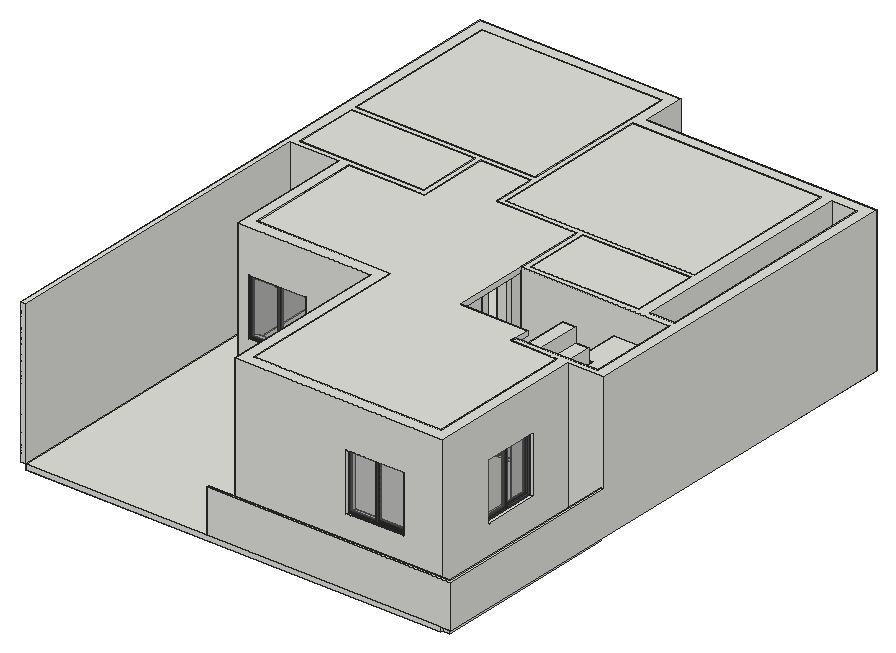
# SketchUp Ruby script. Lengths in inches.
U = 1.inch
M = Sketchup.active_model
def pt(a) = Geom::Point3d.new(a.map { |v| v * U })
def face(e, loops, mat)
  f = e.add_face(loops[0].map { |a| pt(a) })
  loops[1..].each { |l| e.add_face(l.map { |a| pt(a) }).erase! }
  f.material = f.back_material = mat if mat
  f
end
# faces: each face lists its corners as indices into pts; further lists are holes
def faces(e, pts, list, mat = nil) = list.each { |f| face(e, (f[0].is_a?(Array) ? f : [f]).map { |l| l.map { |i| pts[i] } }, mat) }
# xy, xz, yz: faces in a plane at the given z, y or x. An outline is a flat list of corners, or four numbers for a rectangle; further outlines are holes
def ring(l) = l.size == 4 ? [[l[0], l[1]], [l[2], l[1]], [l[2], l[3]], [l[0], l[3]]] : l.each_slice(2).to_a
def flat(e, list, mat, &to3) = list.each { |f| face(e, (f[0].is_a?(Array) ? f : [f]).map { |l| ring(l).map { |u, v| to3.(u, v) } }, mat) }
def xy(e, z, list, mat = nil) = flat(e, list, mat) { |x, y| [x, y, z] }
def xz(e, y, list, mat = nil) = flat(e, list, mat) { |x, z| [x, y, z] }
def yz(e, x, list, mat = nil) = flat(e, list, mat) { |y, z| [x, y, z] }
def lines(e, pts, list) = list.each { |a, b| e.add_line(pt(pts[a]), pt(pts[b])) }
# prism: a flat outline (further loops are holes) pulled along v
def prism(e, loops, v, mat = nil)
  f = face(e, loops, mat); d = Geom::Vector3d.new(v.map { |x| x * U })
  f.pushpull(f.normal.samedirection?(d) ? d.length : -d.length)
end
def box(e, o, s, mat = nil) = prism(e, [[o, [o[0] + s[0], o[1], o[2]], [o[0] + s[0], o[1] + s[1], o[2]], [o[0], o[1] + s[1], o[2]]]], [0, 0, s[2]], mat)
def at(x, y, z, deg = 0) = Geom::Transformation.translation(pt([x, y, z])) * Geom::Transformation.rotation(ORIGIN, Z_AXIS, deg.degrees)
def axes(o, x, y, z) = Geom::Transformation.new([*x, 0, *y, 0, *z, 0, *pt(o).to_a, 1])
def part(name) = M.definitions.add(name)
# library, detail: a bought-in or finely detailed component or shape, given as its bounding box
def library(name, o, s) = part(name).tap { |d| box(d.entities, o, s) }
def detail(e, o, s) = box(e.add_group.entities, o, s)
def put(e, d, t, mat = nil) = e.add_instance(d, t).tap { |i| i.material = mat if mat }
def group(e, t, mat = nil) = e.add_group.tap { |g| g.transformation = t; g.material = mat if mat }.entities
root = M.entities
M.materials.add("[0099_LightSteelBlue]").color = [176, 196, 222]
M.materials.add("[0135_DarkGray]").color = [81, 81, 81]
M.materials.add("[Translucent Glass Gray]1").color = [128, 128, 128]
M.materials["[Translucent Glass Gray]1"].alpha = 0.15
M.materials.add("[Wood Bamboo]").color = [112, 66, 27]
c1 = library("door58",[0,0,0],[34.0625,4.69,78.29])
c2 = library("Flush door assembly",[0,-5.12,-0.12],[5.12,39.07,81.6])
c3 = library("WP_2073",[15.29,-17.35,0],[14.73,29.14,28.74])
c4 = library("Shower-Trim-Delta-Modern-Monitor_14S_Shower_Trim-T14267-PP",[-3.32,-7.77,-3.94],[6.64,7.77,30.2])
c5 = part("PENTEK_RP Fineline 50S_Sliding_DoorCase_E1")
box(c5.entities,[0,0,0],[1.51,3.66,99.27],"[0135_DarkGray]")
c6 = part("PENTEK_RP Fineline 50S_SlidingDooe_Case_E2")
box(c6.entities,[0,0,0],[96.25,3.66,1.51],"[0135_DarkGray]")
c7 = part("pentek_RP Fineline 50S_SlidingDoor_Case")
put(c7.entities,c5,at(97.76,0,0))
put(c7.entities,c6,at(1.51,0,0))
put(c7.entities,c5,at(0,0,0))
put(c7.entities,c6,at(1.51,0,97.76))
c8 = part("PENTEK_RP Fineline 50S_SlidingDoor_GlazingBead_2")
box(c8.entities,[0,0,0],[0.56,0.59,94.39],"[0135_DarkGray]")
c9 = part("PENTEK_RP Fineline 50S_SlidingDoor_Glass")
box(c9.entities,[0,0,0],[46.58,0.16,94.39],"[Translucent Glass Gray]1")
c10 = part("PENTEK_RP Fineline 50S_SlidingDoor_GlazingBead")
box(c10.entities,[0,0,0],[45.47,0.59,0.56],"[0135_DarkGray]")
c11 = part("PENTEK_RP Fineline 50S_SlidingDoor_Leaf_E1")
prism(c11.entities,[[[0,1.97,0],[1.49,1.97,0],[1.49,1.57,0],[0.93,1.57,0],[0.93,0,0],[0,0,0]]],[0,0,96.25],"[0135_DarkGray]")
c12 = part("PENTEK_RP Fineline 50S_SlidingDoor_Leaf_E2")
xy(c12.entities,0,[[0,0,0,1.57,0.56,1.57,0.56,1.97,46.02,1.97,46.02,1.57,46.58,1.57,46.58,0]],"[0135_DarkGray]")
xy(c12.entities,0.93,[[0,0,46.58,1.57]],"[0135_DarkGray]")
xy(c12.entities,1.49,[[0.56,1.57,46.02,1.97]],"[0135_DarkGray]")
xz(c12.entities,0,[[0,0,46.58,0.93]],"[0135_DarkGray]")
xz(c12.entities,1.57,[[0,0,0.56,0.93],[46.02,0,46.58,0.93],[0.56,0.93,46.02,1.49]],"[0135_DarkGray]")
xz(c12.entities,1.97,[[0.56,0,46.02,1.49]],"[0135_DarkGray]")
yz(c12.entities,0,[[0,0,1.57,0.93]],"[0135_DarkGray]")
yz(c12.entities,0.56,[[1.57,0,1.97,1.49]],"[0135_DarkGray]")
yz(c12.entities,46.02,[[1.57,0,1.97,1.49]],"[0135_DarkGray]")
yz(c12.entities,46.58,[[0,0,1.57,0.93]],"[0135_DarkGray]")
c13 = part("PENTEK_RP Fineline S_SlidingDoor_Leaf1")
put(c13.entities,c8,at(0.93,0,0.93))
put(c13.entities,c8,at(46.96,0,0.93))
put(c13.entities,c9,at(1.49,1.42,0.93))
put(c13.entities,c10,at(1.49,0,0.93))
put(c13.entities,c9,at(1.49,0.59,0.93))
put(c13.entities,c11,at(0,0,0))
put(c13.entities,c11,axes([48.44,0,0],[-1,0,0],[0,1,0],[0,0,1]))
put(c13.entities,c12,axes([0.93,0,96.25],[1,0,0],[0,1,0],[0,0,-1]))
put(c13.entities,c12,at(0.93,0,0))
put(c13.entities,c10,at(1.49,0,94.77))
c14 = part("PENTEK_RP Fineline 50S_SlidingDoor_Leaf2")
put(c14.entities,c9,at(1.49,1.42,0.93))
put(c14.entities,c10,at(1.49,0,94.77))
put(c14.entities,c8,at(46.96,0,0.93))
put(c14.entities,c9,at(1.49,0.59,0.93))
put(c14.entities,c8,at(0.93,0,0.93))
put(c14.entities,c11,at(0,0,0))
put(c14.entities,c11,axes([48.44,0,0],[-1,0,0],[0,1,0],[0,0,1]))
put(c14.entities,c10,at(1.49,0,0.93))
put(c14.entities,c12,axes([0.93,0,96.25],[1,0,0],[0,1,0],[0,0,-1]))
put(c14.entities,c12,at(0.93,0,0))
c15 = part("PENTEK_RP+Fineline+50S_Sliding_Door+(1)")
put(c15.entities,c7,at(0,-1.88,-0.09))
put(c15.entities,c13,at(1.51,-2.27,1.42))
put(c15.entities,c14,at(49.32,-0.3,1.42))
c16 = part("Component\#1")
box(c16.entities,[0,0,0],[16.1,26,0.8])
c17 = part("Component\#2")
box(c17.entities,[0,0,0],[25.87,9.8,0.8])
c18 = part("Component\#3")
box(c18.entities,[0,0,0],[12.93,26,0.8])
c19 = library("Group69",[-16.93,-10.04,-8.23],[33.86,20.08,21.73])
c20 = part("Component\#4")
box(c20.entities,[0,0,0],[13.7,49,0.8])
c21 = part("Component\#5")
box(c21.entities,[0,0,0],[15.4,32.2,0.8])
c22 = part("Component\#6")
box(c22.entities,[0,0,0],[23.2,26,0.8],"[0099_LightSteelBlue]")
c23 = library("Group\#11",[-0.5,-0.5,-0.1],[125,90.5,0.2])
xy(root,-4,[[4.5,0,4.5,435,9,435,9,471,159,471,159,435,351,435,351,240,233,240,233,204,351,204,351,200,283,200,283,164,351,164,351,159.5,357.25,159.5,357.25,2.0625,351,2.0625,351,0]])
xy(root,0,[[4.5,0,4.5,435,9,435,9,471,159,471,159,435,351,435,351,240,227,240,227,204,315,204,315,200,293,200,293,164,351,164,351,159.5,357.25,159.5,357.25,2.0625,351,2.0625,351,0]])
xy(root,12,[[227,204,238,240]])
xy(root,24,[[238,204,249,240]])
xy(root,36,[[249,204,260,240]])
xy(root,48,[[260,204,271,240]])
xy(root,60,[[271,204,282,240]])
xy(root,72,[[282,204,293,240]])
xy(root,84,[[293,204,304,240]])
xy(root,96,[[315,164,351,164,351,240,304,240,304,204,315,204]])
xy(root,108,[[304,164,315,200]])
xy(root,120,[[293,164,304,200]])
xz(root,0,[[4.5,-4,351,0]])
xz(root,2.0625,[[351,-4,357.25,0]])
xz(root,159.5,[[351,-4,357.25,0]])
xz(root,164,[[283,-4,351,0],[293,0,351,0,351,96,315,96,315,108,304,108,304,120,293,120]])
xz(root,200,[[293,0,293,120,304,120,304,108,315,108,315,0]])
xz(root,204,[[227,0,315,0,315,96,304,96,304,84,293,84,293,72,282,72,282,60,271,60,271,48,260,48,260,36,249,36,249,24,238,24,238,12,227,12]])
xz(root,240,[[233,-4,351,0],[227,0,227,12,238,12,238,24,249,24,249,36,260,36,260,48,271,48,271,60,282,60,282,72,293,72,293,84,304,84,304,96,351,96,351,0]])
xz(root,435,[[4.5,-4,9,0],[159,-4,351,0]])
xz(root,471,[[9,-4,159,0]])
yz(root,4.5,[[0,-4,435,0]])
yz(root,9,[[435,-4,471,0]])
yz(root,159,[[435,-4,471,0]])
yz(root,227,[[204,0,240,12]])
yz(root,238,[[204,12,240,24]])
yz(root,249,[[204,24,240,36]])
yz(root,260,[[204,36,240,48]])
yz(root,271,[[204,48,240,60]])
yz(root,282,[[204,60,240,72]])
yz(root,293,[[164,0,200,120],[204,72,240,84]])
yz(root,304,[[204,84,240,96],[164,108,200,120]])
yz(root,315,[[200,0,204,96],[164,96,200,108]])
yz(root,351,[[0,-4,2.0625,0],[159.5,-4,164,0],[200,-4,204,96],[240,-4,435,0],[164,96,240,120]])
yz(root,357.25,[[2.0625,-4,159.5,0]])
put(root,c1,axes([156.6875,167,0],[0,-1.05686,0],[1,0,0],[0,0,1.02]))
put(root,c2,axes([111.88,288.7,0.12],[1,0,0],[0,0.81896,0],[0,0,0.98035]))
put(root,c3,axes([240.57,240.54,-0.55],[0.02117,0.99977,0.0026],[-0.83872,0.01765,0.04289],[0.05099,-0.00368,0.99869]))
put(root,c4,at(321,270.72,69.74,-90))
put(root,c3,axes([18.26,279.57,-0.55],[0.02117,0.99977,0.0026],[-0.83872,0.01765,0.04289],[0.05099,-0.00368,0.99869]))
put(root,c4,at(79.9,334.5,69.74))
put(root,c2,axes([262.8,297.88,0.12],[0,1,0],[-0.81896,0,0],[0,0,0.98035]))
put(root,c15,axes([249,32.69,36.04],[0.48352,0,0],[0,1,0],[0,0,0.48352]))
put(root,c15,axes([54,174.03,36.04],[0.48352,0,0],[0,1,0],[0,0,0.48352]))
put(root,c15,axes([325.32,123.5,36.04],[0,-0.48352,0],[1,0,0],[0,0,0.48352]))
g1 = group(root,at(54,180,0))
prism(g1,[[[25,25,0],[110,25,0],[110,0,0],[0,0,0],[0,96,0],[25,96,0]]],[0,0,4])
g2 = group(root,at(54,180,4))
prism(g2,[[[27,96,0],[27,27,0],[110,27,0],[110,0,0],[0,0,0],[0,96,0]],[[2.35,57.97,0],[21.91,57.97,0],[21.91,90.16,0],[2.35,90.16,0]]],[0,0,28])
put(g2,c16,axes([27,78.9,1],[0,1,0],[0,0,1],[1,0,0]))
put(g2,c16,axes([27,62,1],[0,1,0],[0,0,1],[1,0,0]))
put(g2,c16,axes([27,45.5,1],[0,1,0],[0,0,1],[1,0,0]))
put(g2,c16,axes([27,29,1],[0,1,0],[0,0,1],[1,0,0]))
put(g2,c17,axes([81.93,27,17.2],[-1,0,0],[0,0,1],[0,1,0]))
put(g2,c17,axes([81.93,27,6.8],[-1,0,0],[0,0,1],[0,1,0]))
put(g2,c18,axes([109,27,1],[-1,0,0],[0,0,1],[0,1,0]))
put(g2,c18,axes([95.27,27,1],[-1,0,0],[0,0,1],[0,1,0]))
put(g2,c18,axes([55.27,27,1],[-1,0,0],[0,0,1],[0,1,0]))
put(g2,c18,axes([41.93,27,1],[-1,0,0],[0,0,1],[0,1,0]))
g3 = group(g2,at(81.93,27,1))
box(g3,[-25.87,0,0],[25.87,0.8,5.2])
put(root,c19,at(65.87,254.12,30.8,90))
g4 = group(root,at(103,180,62))
box(g4,[0,0,0],[62,18,51])
put(g4,c20,axes([61,18,1],[-1,0,0],[0,0,1],[0,1,0]))
put(g4,c21,axes([46.7,18,17.8],[-1,0,0],[0,0,1],[0,1,0]))
put(g4,c20,axes([14.7,18,1],[-1,0,0],[0,0,1],[0,1,0]))
put(g4,c21,axes([30.7,18,17.8],[-1,0,0],[0,0,1],[0,1,0]))
g5 = group(g4,at(15.3,2,0),"[Wood Bamboo]")
xy(g5,2,[[2,0,29.4,16]])
xy(g5,15,[[2,0,29.4,16]])
xz(g5,0,[[2,2,29.4,15]])
xz(g5,16,[[[0,0,31.4,17],[2,2,29.4,15]]])
yz(g5,2,[[0,2,16,15]])
yz(g5,29.4,[[0,2,16,15]])
g6 = group(root,at(54,180,85))
box(g6,[0,0,0],[49,18,28])
put(g6,c22,axes([48,18,1],[-1,0,0],[0,0,1],[0,1,0]))
put(g6,c22,axes([24.2,18,1],[-1,0,0],[0,0,1],[0,1,0]))
g7 = group(root,at(9,38,120))
box(g7,[154.5,265,-4],[157.5,132,4])
box(g7,[0,301,-4],[150,132,4])
box(g7,[0,242.5,-4],[103.5,54,4])
box(g7,[222,206.5,-4],[90,54,4])
box(g7,[173,17,-6],[122,87.5,2])
xy(g7,-6,[[[156,0,312,121.5],[172,16,296,105.5]]])
xy(g7,-4,[[156,121.5,156,142,45,142,45,238,108,238,108,296.5,150,296.5,150,260.5,217.5,260.5,217.5,138.49,274,138.49,274,121.5]])
xy(g7,0,[[156,0,312,0,312,121.5,274,121.5,274,138.49,217.5,138.49,217.5,260.5,150,260.5,150,296.5,108,296.5,108,238,45,238,45,142,156,142]])
xz(g7,0,[[156,-6,312,0]])
xz(g7,16,[[172,-6,296,-4]])
xz(g7,105.5,[[172,-6,274,-4],[274,-6,296,-4]])
xz(g7,121.5,[[156,-6,274,-4],[274,-6,312,0]])
xz(g7,138.49,[[217.5,-4,274,0]])
xz(g7,142,[[45,-4,156,0]])
xz(g7,238,[[45,-4,108,0]])
xz(g7,260.5,[[150,-4,217.5,0]])
xz(g7,296.5,[[108,-4,150,0]])
yz(g7,45,[[142,-4,238,0]])
yz(g7,108,[[238,-4,296.5,0]])
yz(g7,150,[[260.5,-4,296.5,0]])
yz(g7,156,[[0,-6,0,0,142,0,142,-4,121.5,-4,121.5,-6]])
yz(g7,172,[[16,-6,105.5,-4]])
yz(g7,217.5,[[138.49,-4,260.5,0]])
yz(g7,274,[[121.5,-4,126,0],[126,-4,138.49,0]])
yz(g7,296,[[16,-6,105.5,-4]])
yz(g7,312,[[0,-6,121.5,0]])
put(g7,c23,at(172,16,-4))
g8 = group(root,at(0,0,0))
xy(g8,0,[[[0,0,0,480,168,480,168,444,360,444,360,0,156,0,156,2.0625,357.25,2.0625,357.25,159.5,330,159.5,330,29,156,29,156,131,165,131,165,38,321,38,321,159.5,282,159.5,282,164,351,164,351,200,222.1875,200,222.1875,204,351,204,351,240,226.5,240,226.5,298.5,203.5,298.5,203.5,303,235,303,235,298.5,231,298.5,231,244.5,321,244.5,321,298.5,267,298.5,267,303,321,303,321,435,163.5,435,163.5,303,167.5,303,167.5,298.5,159,298.5,159,334.5,155,334.5,155,339,159,339,159,471,9,471,9,339,119,339,119,334.5,117,334.5,117,316.5,112.5,316.5,112.5,334.5,9,334.5,9,280.5,112.5,280.5,112.5,284.5,117,284.5,117,276,54,276,54,180,165,180,165,167,156,167,156,171,45,171,45,276,4.5,276,4.5,0],[330,244.5,351,435]]])
xy(g8,36,[[156,0,360,0,360,159.5,357.25,159.5,357.25,2.0625,156,2.0625],[249,29,297,38],[321,75.5,330,123.5],[54,171,102,180]])
xy(g8,80,[[156,131,165,167],[112.5,284.5,117,316.5],[167.5,298.5,203.5,303],[235,298.5,267,303],[119,334.5,155,339]])
xy(g8,84,[[249,29,297,38],[321,75.5,330,123.5],[54,171,102,180]])
xy(g8,120,[[[0,0,4.5,0,4.5,276,45,276,45,171,156,171,156,29,330,29,330,159.5,360,159.5,360,444,168,444,168,480,0,480],[165,38,165,180,54,180,54,276,117,276,117,334.5,159,334.5,159,298.5,226.5,298.5,226.5,240,351,240,351,164,282,164,282,159.5,321,159.5,321,38],[163.5,303,321,435],[9,339,159,471],[9,280.5,112.5,334.5],[231,244.5,321,298.5],[330,244.5,351,435]]])
xz(g8,0,[[0,0,4.5,120],[156,0,360,36]])
xz(g8,2.0625,[[156,0,357.25,36]])
xz(g8,29,[[[156,0,330,120],[249,36,297,84]]])
xz(g8,38,[[[165,0,321,120],[249,36,297,84]]])
xz(g8,75.5,[[321,36,330,84]])
xz(g8,123.5,[[321,36,330,84]])
xz(g8,131,[[156,0,165,80]])
xz(g8,159.5,[[282,0,321,120],[330,0,357.25,0,357.25,36,360,36,360,120,330,120]])
xz(g8,164,[[282,0,351,120]])
xz(g8,167,[[156,0,165,80]])
xz(g8,171,[[[45,0,156,120],[54,36,102,84]]])
xz(g8,180,[[54,0,54,36,102,36,102,84,54,84,54,120,165,120,165,0]])
xz(g8,240,[[226.5,0,351,120]])
xz(g8,244.5,[[231,0,321,120],[330,0,351,120]])
xz(g8,276,[[4.5,0,45,120],[54,0,117,120]])
xz(g8,280.5,[[9,0,112.5,120]])
xz(g8,284.5,[[112.5,0,117,80]])
xz(g8,298.5,[[159,0,167.5,0,167.5,80,203.5,80,203.5,0,226.5,0,226.5,120,159,120],[231,0,235,0,235,80,267,80,267,0,321,0,321,120,231,120]])
xz(g8,303,[[163.5,0,163.5,120,321,120,321,0,267,0,267,80,235,80,235,0,203.5,0,203.5,80,167.5,80,167.5,0]])
xz(g8,316.5,[[112.5,0,117,80]])
xz(g8,334.5,[[9,0,112.5,120],[117,0,119,0,119,80,155,80,155,0,159,0,159,120,117,120]])
xz(g8,339,[[9,0,9,120,159,120,159,0,155,0,155,80,119,80,119,0]])
xz(g8,435,[[163.5,0,321,120],[330,0,351,120]])
xz(g8,444,[[168,0,360,120]])
xz(g8,471,[[9,0,159,120]])
xz(g8,480,[[0,0,168,120]])
yz(g8,0,[[0,0,480,120]])
yz(g8,4.5,[[0,0,276,120]])
yz(g8,9,[[280.5,0,334.5,120],[339,0,471,120]])
yz(g8,45,[[171,0,276,120]])
yz(g8,54,[[180,0,276,0,276,120,180,120,180,84,171,84,171,36,180,36]])
yz(g8,102,[[171,36,180,84]])
yz(g8,112.5,[[280.5,0,280.5,120,334.5,120,334.5,0,316.5,0,316.5,80,284.5,80,284.5,0]])
yz(g8,117,[[276,0,284.5,0,284.5,80,316.5,80,316.5,0,334.5,0,334.5,120,276,120]])
yz(g8,119,[[334.5,0,339,80]])
yz(g8,155,[[334.5,0,339,80]])
yz(g8,156,[[0,0,2.0625,36],[29,0,29,120,171,120,171,0,167,0,167,80,131,80,131,0]])
yz(g8,159,[[298.5,0,334.5,120],[339,0,471,120]])
yz(g8,163.5,[[303,0,435,120]])
yz(g8,165,[[38,0,131,0,131,80,167,80,167,0,180,0,180,120,38,120]])
yz(g8,167.5,[[298.5,0,303,80]])
yz(g8,168,[[444,0,480,120]])
yz(g8,203.5,[[298.5,0,303,80]])
yz(g8,226.5,[[240,0,298.5,120]])
yz(g8,231,[[244.5,0,298.5,120]])
yz(g8,235,[[298.5,0,303,80]])
yz(g8,249,[[29,36,38,84]])
yz(g8,267,[[298.5,0,303,80]])
yz(g8,282,[[159.5,0,164,120]])
yz(g8,297,[[29,36,38,84]])
yz(g8,321,[[[38,0,159.5,120],[75.5,36,123.5,84]],[244.5,0,298.5,120],[303,0,435,120]])
yz(g8,330,[[[29,0,159.5,120],[75.5,36,123.5,84]],[244.5,0,435,120]])
yz(g8,351,[[244.5,0,435,120]])
yz(g8,357.25,[[2.0625,0,159.5,36]])
yz(g8,360,[[0,0,444,0,444,120,159.5,120,159.5,36,0,36]])
